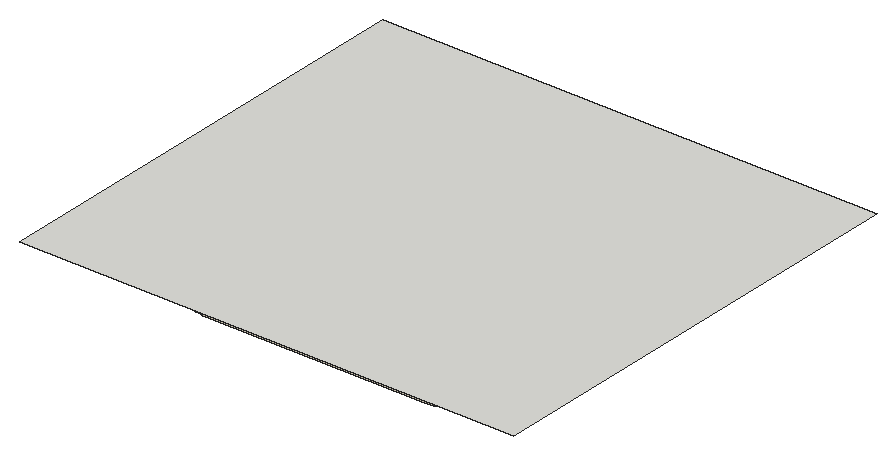
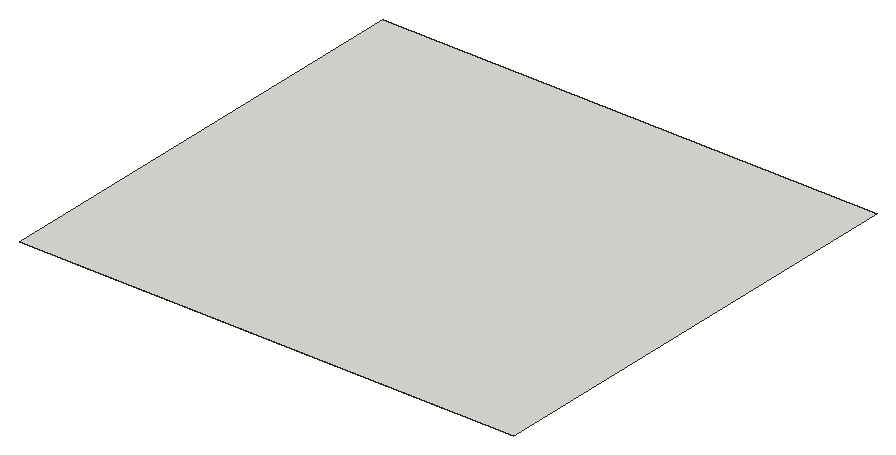
# SketchUp Ruby script. Lengths in inches.
U = 1.inch
M = Sketchup.active_model
def pt(a) = Geom::Point3d.new(a.map { |v| v * U })
def face(e, loops, mat)
  f = e.add_face(loops[0].map { |a| pt(a) })
  loops[1..].each { |l| e.add_face(l.map { |a| pt(a) }).erase! }
  f.material = f.back_material = mat if mat
  f
end
# faces: each face lists its corners as indices into pts; further lists are holes
def faces(e, pts, list, mat = nil) = list.each { |f| face(e, (f[0].is_a?(Array) ? f : [f]).map { |l| l.map { |i| pts[i] } }, mat) }
# xy, xz, yz: faces in a plane at the given z, y or x. An outline is a flat list of corners, or four numbers for a rectangle; further outlines are holes
def ring(l) = l.size == 4 ? [[l[0], l[1]], [l[2], l[1]], [l[2], l[3]], [l[0], l[3]]] : l.each_slice(2).to_a
def flat(e, list, mat, &to3) = list.each { |f| face(e, (f[0].is_a?(Array) ? f : [f]).map { |l| ring(l).map { |u, v| to3.(u, v) } }, mat) }
def xy(e, z, list, mat = nil) = flat(e, list, mat) { |x, y| [x, y, z] }
def xz(e, y, list, mat = nil) = flat(e, list, mat) { |x, z| [x, y, z] }
def yz(e, x, list, mat = nil) = flat(e, list, mat) { |y, z| [x, y, z] }
def lines(e, pts, list) = list.each { |a, b| e.add_line(pt(pts[a]), pt(pts[b])) }
# prism: a flat outline (further loops are holes) pulled along v
def prism(e, loops, v, mat = nil)
  f = face(e, loops, mat); d = Geom::Vector3d.new(v.map { |x| x * U })
  f.pushpull(f.normal.samedirection?(d) ? d.length : -d.length)
end
def box(e, o, s, mat = nil) = prism(e, [[o, [o[0] + s[0], o[1], o[2]], [o[0] + s[0], o[1] + s[1], o[2]], [o[0], o[1] + s[1], o[2]]]], [0, 0, s[2]], mat)
def at(x, y, z, deg = 0) = Geom::Transformation.translation(pt([x, y, z])) * Geom::Transformation.rotation(ORIGIN, Z_AXIS, deg.degrees)
def axes(o, x, y, z) = Geom::Transformation.new([*x, 0, *y, 0, *z, 0, *pt(o).to_a, 1])
def part(name) = M.definitions.add(name)
# library, detail: a bought-in or finely detailed component or shape, given as its bounding box
def library(name, o, s) = part(name).tap { |d| box(d.entities, o, s) }
def detail(e, o, s) = box(e.add_group.entities, o, s)
def put(e, d, t, mat = nil) = e.add_instance(d, t).tap { |i| i.material = mat if mat }
def group(e, t, mat = nil) = e.add_group.tap { |g| g.transformation = t; g.material = mat if mat }.entities
root = M.entities
M.materials.add("0961 AP 7892 PALE IVORY").color = [243, 232, 209]
c1 = library("Group\#16",[-0.5,-0.5,0],[144.26,153.26,1])
xy(root,115.78,[[[76.16,11.37,158.04,11.37,158.99,11.48,159.91,11.61,160.83,11.77,161.75,11.96,162.65,12.17,163.56,12.41,164.45,12.68,165.34,12.98,166.21,13.29,167.08,13.64,167.9375,14.01,168.78,14.41,169.61,14.83,170.44,15.27,171.24,15.74,172.04,16.23,172.8125,16.75,173.58,17.28,174.32,17.84,175.05,18.42,175.76,19.03,176.46,19.65,177.13,20.29,177.79,20.96,178.43,21.64,179.04,22.34,179.64,23.06,180.21,23.8,180.76,24.55,181.29,25.32,181.8,26.1,182.28,26.9,182.74,27.71,183.18,28.54,183.59,29.375,183.98,30.22,184.34,31.08,184.67,31.95,184.98,32.83,185.27,33.72,185.52,34.62,185.76,35.52,185.96,36.43,186.14,37.35,186.29,38.27,186.41,39.2,186.51,40.125,186.58,41.06,186.62,41.99,186.63,42.92,186.63,129,186.62,129.92,186.57,130.84,186.51,131.76,186.41,132.68,186.28,133.59,186.13,134.5,185.95,135.41,185.75,136.31,185.51,137.2,185.26,138.08,184.97,138.96,184.66,139.83,184.32,140.6875,183.96,141.53,183.57,142.37,183.15,143.19,182.71,144,182.25,144.8,181.76,145.59,181.25,146.35,180.72,147.11,180.17,147.84,179.59,148.5625,178.99,149.26,178.375,149.95,177.73,150.61,177.07,151.26,176.4,151.88,175.7,152.49,174.99,153.07,174.25,153.63,173.51,154.17,172.74,154.6875,171.96,155.18,171.17,155.65,170.36,156.1,169.54,156.52,168.71,156.91,167.87,157.29,167.01,157.63,166.15,157.95,165.27,158.25,164.39,158.51,163.5,158.75,162.6,158.97,161.7,159.15,160.79,159.3125,159.88,159.45,158.96,159.55,158.03,159.63,76.18,159.63,75.24,159.56,74.32,159.46,73.4,159.33,72.49,159.18,71.58,159,70.68,158.79,69.78,158.55,68.89,158.29,68.01,158,67.14,157.68,66.28,157.34,65.43,156.97,64.6,156.58,63.77,156.16,62.96,155.71,62.16,155.25,61.37,154.75,60.6,154.24,59.85,153.7,59.11,153.14,58.39,152.56,57.69,151.95,57.01,151.33,56.34,150.68,55.7,150.02,55.07,149.33,54.47,148.63,53.89,147.91,53.33,147.17,52.79,146.42,52.28,145.65,51.79,144.86,51.32,144.0625,50.88,143.25,50.46,142.42,50.07,141.58,49.7,140.73,49.36,139.87,49.05,139,48.76,138.12,48.5,137.23,48.26,136.34,48.05,135.43,47.875,134.53,47.72,133.61,47.59,132.7,47.5,131.77,47.43,130.85,47.39,129.93,47.37,129,47.37,43.85,47.39,42.9,47.43,41.95,47.49,41.01,47.59,40.07,47.71,39.125,47.86,38.1875,48.04,37.26,48.25,36.33,48.48,35.41,48.74,34.5,49.02,33.59,49.33,32.7,49.67,31.8125,50.03,30.93,50.42,30.07,50.83,29.21,51.26,28.37,51.72,27.54,52.21,26.73,52.72,25.93,53.25,25.14,53.8,24.37,54.375,23.62,54.97,22.88,55.59,22.16,56.23,21.46,56.89,20.78,57.57,20.12,58.27,19.47,58.98,18.85,59.71,18.25,60.47,17.67,61.23,17.11,62.02,16.58,62.8125,16.07,63.625,15.58,64.45,15.11,65.29,14.67,66.14,14.25,67.01,13.86,67.88,13.5,68.77,13.15,69.66,12.84,70.5625,12.55,71.48,12.29,72.39,12.05,73.32,11.84,74.25,11.66,75.18,11.5],[76.2,12,75.28,12.125,74.36,12.28,73.45,12.46,72.54,12.66,71.64,12.9,70.75,13.15,69.86,13.4375,68.98,13.75,68.12,14.08,67.26,14.44,66.41,14.82,65.58,15.23,64.75,15.67,63.94,16.12,63.15,16.6,62.36,17.1,61.6,17.63,60.84,18.18,60.11,18.74,59.39,19.33,58.6875,19.94,58,20.57,57.34,21.22,56.69,21.89,56.0625,22.58,55.46,23.29,54.87,24.01,54.31,24.75,53.76,25.5,53.24,26.27,52.75,27.06,52.27,27.86,51.82,28.67,51.39,29.5,50.99,30.33,50.61,31.18,50.25,32.04,49.92,32.91,49.62,33.79,49.34,34.68,49.09,35.57,48.86,36.48,48.66,37.38,48.49,38.3,48.34,39.22,48.22,40.14,48.12,41.0625,48.06,41.99,48.01,42.92,48,43.85,48,129,48.01,129.91,48.06,130.8125,48.125,131.72,48.22,132.62,48.34,133.52,48.49,134.41,48.67,135.3,48.875,136.1875,49.1,137.0625,49.36,137.93,49.64,138.8,49.95,139.65,50.28,140.49,50.64,141.32,51.03,142.15,51.4375,142.96,51.87,143.75,52.33,144.54,52.81,145.31,53.3125,146.06,53.84,146.8,54.39,147.52,54.96,148.23,55.55,148.92,56.16,149.59,56.79,150.24,57.4375,150.87,58.11,151.48,58.8,152.07,59.5,152.64,60.22,153.19,60.96,153.72,61.71,154.23,62.48,154.71,63.27,155.17,64.0625,155.6,64.87,156.01,65.69,156.4,66.52,156.76,67.37,157.09,68.22,157.4,69.08,157.6875,69.95,157.94,70.83,158.17,71.71,158.38,72.6,158.56,73.5,158.71,74.39,158.83,75.3,158.93,76.2,159,158,159,158.9,158.92,159.8,158.82,160.69,158.69,161.58,158.54,162.47,158.35,163.34,158.14,164.22,157.91,165.08,157.65,165.9375,157.36,166.78,157.04,167.62,156.71,168.45,156.34,169.26,155.95,170.07,155.54,170.86,155.1,171.63,154.64,172.4,154.16,173.15,153.65,173.88,153.125,174.59,152.58,175.29,152.01,175.98,151.41,176.64,150.8,177.29,150.17,177.91,149.52,178.52,148.85,179.1,148.16,179.67,147.46,180.21,146.74,180.73,146,181.23,145.25,181.71,144.48,182.16,143.7,182.59,142.9,183,142.1,183.38,141.28,183.74,140.45,184.07,139.61,184.375,138.76,184.65,137.9,184.91,137.03,185.14,136.16,185.34,135.28,185.51,134.39,185.66,133.5,185.78,132.6,185.88,131.71,185.95,130.81,185.99,129.9,186,129,186,42.92,185.99,42.01,185.95,41.09,185.88,40.18,185.78,39.27,185.66,38.36,185.52,37.46,185.34,36.5625,185.14,35.67,184.92,34.78,184.66,33.91,184.39,33.03,184.08,32.17,183.75,31.32,183.4,30.47,183.02,29.64,182.62,28.82,182.19,28.01,181.74,27.22,181.27,26.43,180.77,25.67,180.25,24.91,179.71,24.18,179.15,23.45,178.5625,22.75,177.96,22.0625,177.34,21.39,176.69,20.74,176.03,20.11,175.35,19.5,174.65,18.91,173.9375,18.34,173.21,17.79,172.46,17.27,171.7,16.76,170.92,16.28,170.13,15.82,169.32,15.38,168.51,14.97,167.68,14.58,166.84,14.22,165.99,13.88,165.13,13.57,164.26,13.28,163.38,13.02,162.5,12.78,161.61,12.57,160.71,12.39,159.8125,12.23,158.91,12.1,158,12]]],"0961 AP 7892 PALE IVORY")
xy(root,116.78,[[[75.91,7.74,158.24,7.74,159.45,7.88,160.48,8.03,161.51,8.21,162.53,8.41,163.54,8.65,164.54,8.92,165.54,9.22,166.53,9.55,167.51,9.9,168.47,10.29,169.43,10.7,170.37,11.14,171.3,11.61,172.21,12.1,173.11,12.625,173.99,13.17,174.86,13.75,175.71,14.35,176.54,14.97,177.36,15.62,178.15,16.29,178.92,16.99,179.68,17.7,180.41,18.44,181.12,19.2,181.8,19.98,182.47,20.79,183.11,21.61,183.72,22.44,184.3125,23.3,184.88,24.17,185.42,25.0625,185.93,25.97,186.41,26.89,186.87,27.82,187.3,28.77,187.7,29.73,188.08,30.7,188.42,31.68,188.74,32.67,189.03,33.67,189.29,34.68,189.51,35.69,189.71,36.71,189.88,37.74,190.02,38.77,190.12,39.8,190.2,40.84,190.24,41.88,190.26,42.89,190.26,129.03,190.24,130.03,190.2,131.0625,190.12,132.09,190.01,133.11,189.875,134.14,189.7,135.15,189.5,136.17,189.27,137.17,189.01,138.17,188.72,139.16,188.4,140.14,188.05,141.11,187.68,142.07,187.27,143.02,186.83,143.95,186.37,144.87,185.88,145.78,185.36,146.67,184.82,147.55,184.25,148.41,183.65,149.25,183.03,150.07,182.39,150.875,181.72,151.66,181.03,152.43,180.3125,153.17,179.58,153.89,178.82,154.59,178.04,155.26,177.24,155.92,176.42,156.54,175.59,157.15,174.73,157.73,173.86,158.28,172.97,158.8,172.07,159.3,171.15,159.77,170.22,160.22,169.28,160.63,168.32,161.02,167.35,161.375,166.375,161.7,165.39,162,164.39,162.27,163.39,162.51,162.38,162.72,161.37,162.9,160.35,163.05,159.32,163.16,158.18,163.26,76.04,163.26,74.9,163.17,73.875,163.0625,72.85,162.92,71.83,162.75,70.8125,162.54,69.8,162.31,68.8,162.05,67.81,161.75,66.83,161.43,65.85,161.07,64.89,160.69,63.94,160.28,63,159.84,62.08,159.37,61.17,158.875,60.28,158.35,59.4,157.8,58.54,157.22,57.7,156.62,56.87,156,56.07,155.34,55.28,154.67,54.52,153.97,53.77,153.25,53.05,152.5,52.36,151.74,51.68,150.95,51.03,150.15,50.41,149.32,49.8,148.48,49.23,147.62,48.68,146.74,48.16,145.84,47.66,144.93,47.2,144.01,46.76,143.07,46.35,142.12,45.97,141.16,45.61,140.18,45.29,139.2,45,138.21,44.74,137.21,44.5,136.2,44.3,135.18,44.13,134.16,43.99,133.13,43.88,132.1,43.8,131.07,43.76,130.04,43.74,129.03,43.74,43.82,43.76,42.8,43.8,41.74,43.88,40.69,43.99,39.65,44.12,38.6,44.29,37.5625,44.49,36.53,44.71,35.5,44.97,34.48,45.26,33.46,45.57,32.46,45.92,31.46,46.29,30.48,46.69,29.5,47.12,28.54,47.58,27.59,48.07,26.66,48.58,25.73,49.12,24.83,49.68,23.9375,50.27,23.07,50.88,22.21,51.52,21.375,52.1875,20.56,52.875,19.76,53.58,18.98,54.32,18.22,55.07,17.48,55.84,16.77,56.64,16.08,57.45,15.41,58.29,14.77,59.14,14.15,60.01,13.55,60.9,12.98,61.8,12.44,62.72,11.92,63.65,11.43,64.6,10.97,65.56,10.53,66.53,10.13,67.51,9.75,68.5,9.4,69.51,9.08,70.52,8.79,71.54,8.52,72.57,8.29,73.6,8.09,74.64,7.91],[75.95,8.37,74.73,8.54,73.71,8.71,72.7,8.91,71.6875,9.14,70.69,9.39,69.69,9.68,68.7,10,67.73,10.34,66.76,10.71,65.81,11.11,64.86,11.54,63.93,11.99,63.02,12.48,62.12,12.98,61.23,13.52,60.36,14.08,59.5,14.66,58.67,15.27,57.85,15.9,57.05,16.56,56.26,17.24,55.5,17.94,54.76,18.66,54.04,19.41,53.35,20.17,52.67,20.96,52.02,21.76,51.39,22.59,50.79,23.43,50.21,24.28,49.65,25.16,49.125,26.05,48.62,26.95,48.14,27.87,47.69,28.81,47.27,29.75,46.88,30.71,46.51,31.68,46.17,32.65,45.86,33.64,45.58,34.64,45.33,35.64,45.1,36.65,44.91,37.67,44.75,38.69,44.61,39.72,44.51,40.75,44.43,41.78,44.39,42.82,44.37,43.82,44.37,129.03,44.39,130.02,44.43,131.03,44.51,132.05,44.62,133.06,44.75,134.0625,44.92,135.07,45.12,136.0625,45.35,137.05,45.61,138.04,45.89,139.01,46.21,139.98,46.56,140.93,46.93,141.88,47.33,142.8125,47.76,143.73,48.22,144.64,48.71,145.53,49.22,146.41,49.76,147.28,50.32,148.12,50.91,148.95,51.53,149.76,52.17,150.55,52.83,151.32,53.51,152.07,54.22,152.8,54.95,153.51,55.7,154.2,56.47,154.86,57.26,155.5,58.07,156.12,58.9,156.71,59.74,157.27,60.6,157.8125,61.48,158.33,62.37,158.8125,63.28,159.27,64.2,159.7,65.13,160.11,66.08,160.48,67.03,160.83,68,161.15,68.97,161.4375,69.95,161.7,70.95,161.93,71.94,162.13,72.94,162.3,73.95,162.4375,74.96,162.55,76.0625,162.63,158.15,162.63,159.26,162.54,160.26,162.42,161.27,162.28,162.26,162.1,163.25,161.9,164.24,161.66,165.22,161.4,166.19,161.1,167.14,160.78,168.09,160.43,169.03,160.05,169.96,159.64,170.87,159.21,171.77,158.74,172.66,158.26,173.53,157.74,174.39,157.2,175.22,156.63,176.05,156.04,176.85,155.42,177.63,154.78,178.4,154.12,179.14,153.43,179.86,152.72,180.57,152,181.25,151.25,181.9,150.47,182.54,149.68,183.15,148.875,183.73,148.05,184.29,147.21,184.82,146.35,185.33,145.47,185.8125,144.58,186.27,143.68,186.69,142.76,187.09,141.83,187.46,140.89,187.81,139.93,188.12,138.97,188.41,138,188.66,137.02,188.89,136.03,189.08,135.04,189.25,134.04,189.39,133.04,189.49,132.03,189.57,131.02,189.62,130.01,189.63,129.03,189.63,42.89,189.62,41.9,189.57,40.88,189.5,39.86,189.39,38.84,189.26,37.83,189.09,36.82,188.9,35.82,188.67,34.82,188.42,33.83,188.14,32.85,187.83,31.88,187.49,30.92,187.12,29.96,186.73,29.02,186.3,28.09,185.85,27.17,185.375,26.27,184.87,25.38,184.34,24.51,183.79,23.65,183.21,22.81,182.6,21.99,181.98,21.18,181.33,20.39,180.65,19.625,179.95,18.88,179.24,18.15,178.5,17.45,177.74,16.77,176.96,16.11,176.16,15.47,175.34,14.86,174.51,14.27,173.65,13.7,172.79,13.17,171.9,12.65,171,12.17,170.09,11.71,169.17,11.27,168.23,10.87,167.28,10.49,166.32,10.14,165.35,9.82,164.37,9.53,163.39,9.26,162.39,9.03,161.39,8.82,160.38,8.65,159.375,8.5,158.21,8.37]]],"0961 AP 7892 PALE IVORY")
xz(root,7.74,[[75.91,113.78,158.24,116.78]],"0961 AP 7892 PALE IVORY")
xz(root,8.37,[[75.95,113.78,158.21,116.78]],"0961 AP 7892 PALE IVORY")
yz(root,43.74,[[43.82,113.78,129.03,116.78]],"0961 AP 7892 PALE IVORY")
yz(root,44.37,[[43.82,113.78,129.03,116.78]],"0961 AP 7892 PALE IVORY")
yz(root,189.63,[[42.89,113.78,129.03,116.78]],"0961 AP 7892 PALE IVORY")
yz(root,190.26,[[42.89,113.78,129.03,116.78]],"0961 AP 7892 PALE IVORY")
p = [[74.64,7.91,113.78],[75.91,7.74,113.78],[75.91,7.74,116.78],[74.64,7.91,116.78],[158.24,7.74,113.78],[159.45,7.88,113.78],
  [159.45,7.88,116.78],[158.24,7.74,116.78],[73.6,8.09,113.78],[73.6,8.09,116.78],[160.48,8.03,113.78],[160.48,8.03,116.78],
  [161.51,8.21,113.78],[161.51,8.21,116.78],[72.57,8.29,113.78],[72.57,8.29,116.78],[162.53,8.41,113.78],[162.53,8.41,116.78],
  [71.54,8.52,113.78],[71.54,8.52,116.78],[75.95,8.37,113.78],[74.73,8.54,113.78],[74.73,8.54,116.78],[75.95,8.37,116.78],
  [159.375,8.5,113.78],[158.21,8.37,113.78],[158.21,8.37,116.78],[159.375,8.5,116.78],[163.54,8.65,113.78],[163.54,8.65,116.78],
  [70.52,8.79,113.78],[70.52,8.79,116.78],[73.71,8.71,113.78],[73.71,8.71,116.78],[160.38,8.65,113.78],[160.38,8.65,116.78],
  [161.39,8.82,113.78],[161.39,8.82,116.78],[72.7,8.91,113.78],[72.7,8.91,116.78],[164.54,8.92,113.78],[164.54,8.92,116.78],
  [69.51,9.08,113.78],[69.51,9.08,116.78],[162.39,9.03,113.78],[162.39,9.03,116.78],[71.6875,9.14,113.78],[71.6875,9.14,116.78],
  [165.54,9.22,113.78],[165.54,9.22,116.78],[163.39,9.26,113.78],[163.39,9.26,116.78],[68.5,9.4,113.78],[68.5,9.4,116.78],
  [70.69,9.39,113.78],[70.69,9.39,116.78],[166.53,9.55,113.78],[166.53,9.55,116.78],[164.37,9.53,113.78],[164.37,9.53,116.78],
  [67.51,9.75,113.78],[67.51,9.75,116.78],[69.69,9.68,113.78],[69.69,9.68,116.78],[165.35,9.82,113.78],[165.35,9.82,116.78],
  [167.51,9.9,113.78],[167.51,9.9,116.78],[66.53,10.13,113.78],[66.53,10.13,116.78],[68.7,10,113.78],[68.7,10,116.78],
  [166.32,10.14,113.78],[166.32,10.14,116.78],[168.47,10.29,113.78],[168.47,10.29,116.78],[67.73,10.34,113.78],[67.73,10.34,116.78],
  [65.56,10.53,113.78],[65.56,10.53,116.78],[167.28,10.49,113.78],[167.28,10.49,116.78],[66.76,10.71,113.78],[66.76,10.71,116.78],
  [169.43,10.7,113.78],[169.43,10.7,116.78],[64.6,10.97,113.78],[64.6,10.97,116.78],[168.23,10.87,113.78],[168.23,10.87,116.78],
  [65.81,11.11,113.78],[65.81,11.11,116.78],[170.37,11.14,113.78],[170.37,11.14,116.78],[169.17,11.27,113.78],[169.17,11.27,116.78],
  [63.65,11.43,113.78],[63.65,11.43,116.78],[64.86,11.54,113.78],[64.86,11.54,116.78],[171.3,11.61,113.78],[171.3,11.61,116.78],
  [170.09,11.71,113.78],[170.09,11.71,116.78],[62.72,11.92,113.78],[62.72,11.92,116.78],[63.93,11.99,113.78],[63.93,11.99,116.78],
  [172.21,12.1,113.78],[172.21,12.1,116.78],[171,12.17,113.78],[171,12.17,116.78],[61.8,12.44,113.78],[61.8,12.44,116.78],
  [63.02,12.48,113.78],[63.02,12.48,116.78],[173.11,12.625,113.78],[173.11,12.625,116.78],[171.9,12.65,113.78],[171.9,12.65,116.78],
  [60.9,12.98,113.78],[60.9,12.98,116.78],[62.12,12.98,113.78],[62.12,12.98,116.78],[173.99,13.17,113.78],[173.99,13.17,116.78],
  [172.79,13.17,113.78],[172.79,13.17,116.78],[60.01,13.55,113.78],[60.01,13.55,116.78],[61.23,13.52,113.78],[61.23,13.52,116.78],
  [173.65,13.7,113.78],[173.65,13.7,116.78],[174.86,13.75,113.78],[174.86,13.75,116.78],[60.36,14.08,113.78],[60.36,14.08,116.78],
  [59.14,14.15,113.78],[59.14,14.15,116.78],[174.51,14.27,113.78],[174.51,14.27,116.78],[175.71,14.35,113.78],[175.71,14.35,116.78],
  [58.29,14.77,113.78],[58.29,14.77,116.78],[59.5,14.66,113.78],[59.5,14.66,116.78],[175.34,14.86,113.78],[175.34,14.86,116.78],
  [176.54,14.97,113.78],[176.54,14.97,116.78],[58.67,15.27,113.78],[58.67,15.27,116.78],[57.45,15.41,113.78],[57.45,15.41,116.78],
  [176.16,15.47,113.78],[176.16,15.47,116.78],[177.36,15.62,113.78],[177.36,15.62,116.78],[57.85,15.9,113.78],[57.85,15.9,116.78],
  [56.64,16.08,113.78],[56.64,16.08,116.78],[176.96,16.11,113.78],[176.96,16.11,116.78],[178.15,16.29,113.78],[178.15,16.29,116.78],
  [57.05,16.56,113.78],[57.05,16.56,116.78],[55.84,16.77,113.78],[55.84,16.77,116.78],[177.74,16.77,113.78],[177.74,16.77,116.78],
  [178.92,16.99,113.78],[178.92,16.99,116.78],[56.26,17.24,113.78],[56.26,17.24,116.78],[55.07,17.48,113.78],[55.07,17.48,116.78],
  [178.5,17.45,113.78],[178.5,17.45,116.78],[179.68,17.7,113.78],[179.68,17.7,116.78],[55.5,17.94,113.78],[55.5,17.94,116.78],
  [179.24,18.15,113.78],[179.24,18.15,116.78],[54.32,18.22,113.78],[54.32,18.22,116.78],[180.41,18.44,113.78],[180.41,18.44,116.78],
  [54.76,18.66,113.78],[54.76,18.66,116.78],[53.58,18.98,113.78],[53.58,18.98,116.78],[179.95,18.88,113.78],[179.95,18.88,116.78],
  [181.12,19.2,113.78],[181.12,19.2,116.78],[54.04,19.41,113.78],[54.04,19.41,116.78],[180.65,19.625,113.78],[180.65,19.625,116.78],
  [52.875,19.76,113.78],[52.875,19.76,116.78],[181.8,19.98,113.78],[181.8,19.98,116.78],[53.35,20.17,113.78],[53.35,20.17,116.78],
  [181.33,20.39,113.78],[181.33,20.39,116.78],[52.1875,20.56,113.78],[52.1875,20.56,116.78],[182.47,20.79,113.78],[182.47,20.79,116.78],
  [52.67,20.96,113.78],[52.67,20.96,116.78],[181.98,21.18,113.78],[181.98,21.18,116.78],[51.52,21.375,113.78],[51.52,21.375,116.78],
  [183.11,21.61,113.78],[183.11,21.61,116.78],[52.02,21.76,113.78],[52.02,21.76,116.78],[182.6,21.99,113.78],[182.6,21.99,116.78],
  [50.88,22.21,113.78],[50.88,22.21,116.78],[183.72,22.44,113.78],[183.72,22.44,116.78],[51.39,22.59,113.78],[51.39,22.59,116.78],
  [183.21,22.81,113.78],[183.21,22.81,116.78],[50.27,23.07,113.78],[50.27,23.07,116.78],[184.3125,23.3,113.78],[184.3125,23.3,116.78],
  [50.79,23.43,113.78],[50.79,23.43,116.78],[183.79,23.65,113.78],[183.79,23.65,116.78],[49.68,23.9375,113.78],[49.68,23.9375,116.78],
  [184.88,24.17,113.78],[184.88,24.17,116.78],[50.21,24.28,113.78],[50.21,24.28,116.78],[184.34,24.51,113.78],[184.34,24.51,116.78],
  [49.12,24.83,113.78],[49.12,24.83,116.78],[185.42,25.0625,113.78],[185.42,25.0625,116.78],[49.65,25.16,113.78],[49.65,25.16,116.78],
  [184.87,25.38,113.78],[184.87,25.38,116.78],[48.58,25.73,113.78],[48.58,25.73,116.78],[185.93,25.97,113.78],[185.93,25.97,116.78],
  [49.125,26.05,113.78],[49.125,26.05,116.78],[185.375,26.27,113.78],[185.375,26.27,116.78],[48.07,26.66,113.78],[48.07,26.66,116.78],
  [48.62,26.95,113.78],[48.62,26.95,116.78],[186.41,26.89,113.78],[186.41,26.89,116.78],[185.85,27.17,113.78],[185.85,27.17,116.78],
  [47.58,27.59,113.78],[47.58,27.59,116.78],[186.87,27.82,113.78],[186.87,27.82,116.78],[48.14,27.87,113.78],[48.14,27.87,116.78],
  [186.3,28.09,113.78],[186.3,28.09,116.78],[47.12,28.54,113.78],[47.12,28.54,116.78],[187.3,28.77,113.78],[187.3,28.77,116.78],
  [47.69,28.81,113.78],[47.69,28.81,116.78],[186.73,29.02,113.78],[186.73,29.02,116.78],[46.69,29.5,113.78],[46.69,29.5,116.78],
  [47.27,29.75,113.78],[47.27,29.75,116.78],[187.7,29.73,113.78],[187.7,29.73,116.78],[187.12,29.96,113.78],[187.12,29.96,116.78],
  [46.29,30.48,113.78],[46.29,30.48,116.78],[188.08,30.7,113.78],[188.08,30.7,116.78],[46.88,30.71,113.78],[46.88,30.71,116.78],
  [187.49,30.92,113.78],[187.49,30.92,116.78],[45.92,31.46,113.78],[45.92,31.46,116.78],[46.51,31.68,113.78],[46.51,31.68,116.78],
  [188.42,31.68,113.78],[188.42,31.68,116.78],[187.83,31.88,113.78],[187.83,31.88,116.78],[45.57,32.46,113.78],[45.57,32.46,116.78],
  [46.17,32.65,113.78],[46.17,32.65,116.78],[188.74,32.67,113.78],[188.74,32.67,116.78],[188.14,32.85,113.78],[188.14,32.85,116.78],
  [45.26,33.46,113.78],[45.26,33.46,116.78],[45.86,33.64,113.78],[45.86,33.64,116.78],[189.03,33.67,113.78],[189.03,33.67,116.78],
  [188.42,33.83,113.78],[188.42,33.83,116.78],[44.97,34.48,113.78],[44.97,34.48,116.78],[45.58,34.64,113.78],[45.58,34.64,116.78],
  [189.29,34.68,113.78],[189.29,34.68,116.78],[188.67,34.82,113.78],[188.67,34.82,116.78],[44.71,35.5,113.78],[44.71,35.5,116.78],
  [45.33,35.64,113.78],[45.33,35.64,116.78],[189.51,35.69,113.78],[189.51,35.69,116.78],[188.9,35.82,113.78],[188.9,35.82,116.78],
  [44.49,36.53,113.78],[44.49,36.53,116.78],[45.1,36.65,113.78],[45.1,36.65,116.78],[189.71,36.71,113.78],[189.71,36.71,116.78],
  [189.09,36.82,113.78],[189.09,36.82,116.78],[44.29,37.5625,113.78],[44.29,37.5625,116.78],[44.91,37.67,113.78],[44.91,37.67,116.78],
  [189.88,37.74,113.78],[189.88,37.74,116.78],[189.26,37.83,113.78],[189.26,37.83,116.78],[44.12,38.6,113.78],[44.12,38.6,116.78],
  [44.75,38.69,113.78],[44.75,38.69,116.78],[190.02,38.77,113.78],[190.02,38.77,116.78],[189.39,38.84,113.78],[189.39,38.84,116.78],
  [43.99,39.65,113.78],[43.99,39.65,116.78],[44.61,39.72,113.78],[44.61,39.72,116.78],[189.5,39.86,113.78],[189.5,39.86,116.78],
  [190.12,39.8,113.78],[190.12,39.8,116.78],[43.88,40.69,113.78],[43.88,40.69,116.78],[44.51,40.75,113.78],[44.51,40.75,116.78],
  [190.2,40.84,113.78],[190.2,40.84,116.78],[189.57,40.88,113.78],[189.57,40.88,116.78],[43.8,41.74,113.78],[43.8,41.74,116.78],
  [44.43,41.78,113.78],[44.43,41.78,116.78],[190.24,41.88,113.78],[190.24,41.88,116.78],[189.62,41.9,113.78],[189.62,41.9,116.78],
  [43.76,42.8,113.78],[43.76,42.8,116.78],[44.39,42.82,113.78],[44.39,42.82,116.78],[189.63,42.89,113.78],[189.63,42.89,116.78],
  [190.26,42.89,113.78],[190.26,42.89,116.78],[43.74,43.82,113.78],[43.74,43.82,116.78],[44.37,43.82,113.78],[44.37,43.82,116.78],
  [43.76,130.04,113.78],[43.74,129.03,113.78],[43.74,129.03,116.78],[43.76,130.04,116.78],[44.37,129.03,113.78],[44.39,130.02,113.78],
  [44.39,130.02,116.78],[44.37,129.03,116.78],[189.62,130.01,113.78],[189.63,129.03,113.78],[189.63,129.03,116.78],[189.62,130.01,116.78],
  [190.26,129.03,113.78],[190.24,130.03,113.78],[190.24,130.03,116.78],[190.26,129.03,116.78]]
faces(root,p,[[0,1,2,3],[4,5,6,7],[8,0,3,9],[5,10,11,6],[10,12,13,11],[14,8,9,15],[12,16,17,13],[18,14,15,19],
  [20,21,22,23],[24,25,26,27],[16,28,29,17],[30,18,19,31],[21,32,33,22],[34,24,27,35],[36,34,35,37],[32,38,39,33],
  [28,40,41,29],[42,30,31,43],[44,36,37,45],[38,46,47,39],[40,48,49,41],[50,44,45,51],[52,42,43,53],[46,54,55,47],
  [48,56,57,49],[58,50,51,59],[60,52,53,61],[54,62,63,55],[64,58,59,65],[56,66,67,57],[68,60,61,69],[62,70,71,63],
  [72,64,65,73],[66,74,75,67],[70,76,77,71],[78,68,69,79],[80,72,73,81],[76,82,83,77],[74,84,85,75],[86,78,79,87],
  [88,80,81,89],[82,90,91,83],[84,92,93,85],[94,88,89,95],[96,86,87,97],[90,98,99,91],[92,100,101,93],[102,94,95,103],
  [104,96,97,105],[98,106,107,99],[100,108,109,101],[110,102,103,111],[112,104,105,113],[106,114,115,107],[108,116,117,109],[118,110,111,119],
  [120,112,113,121],[114,122,123,115],[116,124,125,117],[126,118,119,127],[128,120,121,129],[122,130,131,123],[132,126,127,133],[124,134,135,125],
  [130,136,137,131],[138,128,129,139],[140,132,133,141],[134,142,143,135],[144,138,139,145],[136,146,147,137],[148,140,141,149],[142,150,151,143],
  [146,152,153,147],[154,144,145,155],[156,148,149,157],[150,158,159,151],[152,160,161,153],[162,154,155,163],[164,156,157,165],[158,166,167,159],
  [160,168,169,161],[170,162,163,171],[172,164,165,173],[166,174,175,167],[168,176,177,169],[178,170,171,179],[180,172,173,181],[174,182,183,175],
  [176,184,185,177],[186,180,181,187],[188,178,179,189],[182,190,191,183],[184,192,193,185],[194,188,189,195],[196,186,187,197],[190,198,199,191],
  [192,200,201,193],[202,196,197,203],[204,194,195,205],[198,206,207,199],[200,208,209,201],[210,202,203,211],[212,204,205,213],[206,214,215,207],
  [208,216,217,209],[218,210,211,219],[220,212,213,221],[214,222,223,215],[216,224,225,217],[226,218,219,227],[228,220,221,229],[222,230,231,223],
  [224,232,233,225],[234,226,227,235],[236,228,229,237],[230,238,239,231],[232,240,241,233],[242,234,235,243],[244,236,237,245],[238,246,247,239],
  [240,248,249,241],[250,242,243,251],[252,244,245,253],[246,254,255,247],[248,256,257,249],[258,250,251,259],[260,252,253,261],[254,262,263,255],
  [256,264,265,257],[266,258,259,267],[268,260,261,269],[264,270,271,265],[262,272,273,263],[274,266,267,275],[276,268,269,277],[272,278,279,273],
  [270,280,281,271],[282,274,275,283],[284,276,277,285],[278,286,287,279],[280,288,289,281],[290,282,283,291],[292,284,285,293],[288,294,295,289],
  [286,296,297,287],[298,290,291,299],[300,292,293,301],[296,302,303,297],[294,304,305,295],[306,298,299,307],[308,300,301,309],[304,310,311,305],
  [302,312,313,303],[314,306,307,315],[316,308,309,317],[310,318,319,311],[312,320,321,313],[322,314,315,323],[324,316,317,325],[318,326,327,319],
  [320,328,329,321],[330,322,323,331],[332,324,325,333],[326,334,335,327],[328,336,337,329],[338,330,331,339],[340,332,333,341],[334,342,343,335],
  [336,344,345,337],[346,338,339,347],[348,340,341,349],[342,350,351,343],[344,352,353,345],[354,346,347,355],[356,348,349,357],[350,358,359,351],
  [352,360,361,353],[362,354,355,363],[364,356,357,365],[358,366,367,359],[360,368,369,361],[370,362,363,371],[372,364,365,373],[366,374,375,367],
  [376,370,371,377],[368,378,379,369],[380,372,373,381],[374,382,383,375],[378,384,385,379],[386,376,377,387],[388,380,381,389],[382,390,391,383],
  [384,392,393,385],[394,386,387,395],[396,388,389,397],[390,398,399,391],[400,394,395,401],[392,402,403,393],[404,396,397,405],[398,406,407,399],
  [408,409,410,411],[412,413,414,415],[416,417,418,419],[420,421,422,423]],"0961 AP 7892 PALE IVORY")
put(root,c1,at(45.37,9.37,113.78),"0961 AP 7892 PALE IVORY")
g1 = group(root,at(12,0,120))
xy(g1,0,[[0,0,186,171]])
